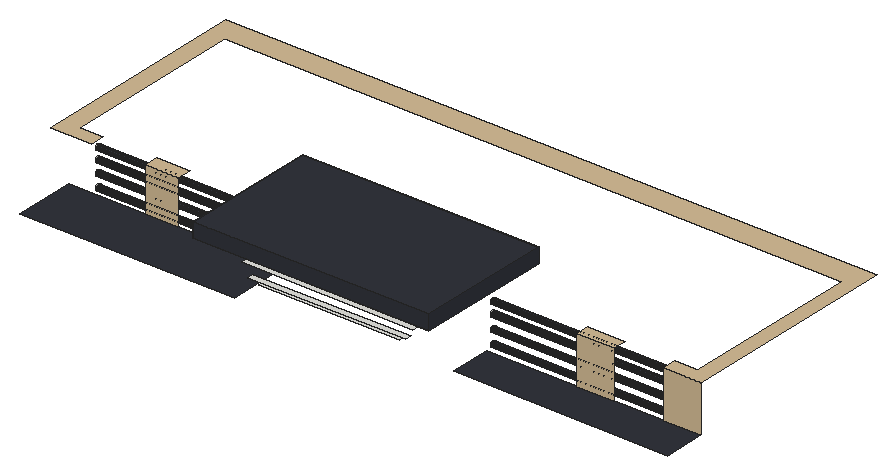
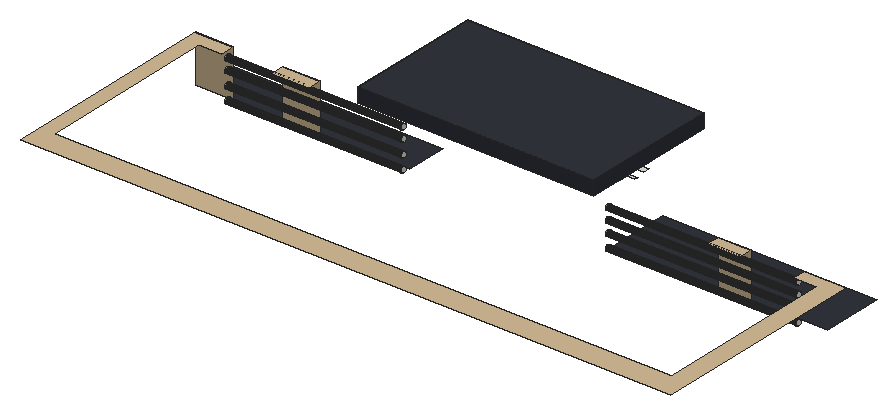
# SketchUp Ruby script. Lengths in inches.
U = 1.inch
M = Sketchup.active_model
def pt(a) = Geom::Point3d.new(a.map { |v| v * U })
def face(e, loops, mat)
  f = e.add_face(loops[0].map { |a| pt(a) })
  loops[1..].each { |l| e.add_face(l.map { |a| pt(a) }).erase! }
  f.material = f.back_material = mat if mat
  f
end
# faces: each face lists its corners as indices into pts; further lists are holes
def faces(e, pts, list, mat = nil) = list.each { |f| face(e, (f[0].is_a?(Array) ? f : [f]).map { |l| l.map { |i| pts[i] } }, mat) }
# xy, xz, yz: faces in a plane at the given z, y or x. An outline is a flat list of corners, or four numbers for a rectangle; further outlines are holes
def ring(l) = l.size == 4 ? [[l[0], l[1]], [l[2], l[1]], [l[2], l[3]], [l[0], l[3]]] : l.each_slice(2).to_a
def flat(e, list, mat, &to3) = list.each { |f| face(e, (f[0].is_a?(Array) ? f : [f]).map { |l| ring(l).map { |u, v| to3.(u, v) } }, mat) }
def xy(e, z, list, mat = nil) = flat(e, list, mat) { |x, y| [x, y, z] }
def xz(e, y, list, mat = nil) = flat(e, list, mat) { |x, z| [x, y, z] }
def yz(e, x, list, mat = nil) = flat(e, list, mat) { |y, z| [x, y, z] }
def lines(e, pts, list) = list.each { |a, b| e.add_line(pt(pts[a]), pt(pts[b])) }
# prism: a flat outline (further loops are holes) pulled along v
def prism(e, loops, v, mat = nil)
  f = face(e, loops, mat); d = Geom::Vector3d.new(v.map { |x| x * U })
  f.pushpull(f.normal.samedirection?(d) ? d.length : -d.length)
end
def box(e, o, s, mat = nil) = prism(e, [[o, [o[0] + s[0], o[1], o[2]], [o[0] + s[0], o[1] + s[1], o[2]], [o[0], o[1] + s[1], o[2]]]], [0, 0, s[2]], mat)
def at(x, y, z, deg = 0) = Geom::Transformation.translation(pt([x, y, z])) * Geom::Transformation.rotation(ORIGIN, Z_AXIS, deg.degrees)
def axes(o, x, y, z) = Geom::Transformation.new([*x, 0, *y, 0, *z, 0, *pt(o).to_a, 1])
def part(name) = M.definitions.add(name)
# library, detail: a bought-in or finely detailed component or shape, given as its bounding box
def library(name, o, s) = part(name).tap { |d| box(d.entities, o, s) }
def detail(e, o, s) = box(e.add_group.entities, o, s)
def put(e, d, t, mat = nil) = e.add_instance(d, t).tap { |i| i.material = mat if mat }
def group(e, t, mat = nil) = e.add_group.tap { |g| g.transformation = t; g.material = mat if mat }.entities
root = M.entities
M.materials.add("[Formica Beige]").color = [211, 187, 149]
M.materials.add("[Formica Laminate Dark]").color = [50, 53, 60]
xy(root,263.9375,[[280.13,426.61,409.38,451.42]],"[Formica Laminate Dark]")
xy(root,265.6875,[[28.78,414.84,157.59,451.42]],"[Formica Laminate Dark]")
xy(root,279.69,[[174.14,412.53,259.2,414.84]])
xy(root,284,[[170.76,408.78,265.76,412.53]])
xy(root,290.79,[[166.89,408.78,270.12,414.84]])
xy(root,292.375,[[17.625,451.42,42.4,451.42,42.4,459.89,28.78,459.89,28.78,568.57,400.54,568.57,400.54,459.89,386.6,459.89,386.6,451.42,409.38,451.42,409.38,583.14,17.625,583.14],[74.87,451.42,94.58,459.89],[334.34,451.42,356.76,459.89]],"[Formica Beige]")
xy(root,305.4375,[[157.59,414.84,280.13,463.02]])
xy(root,305.4375,[[150.71,392.47,292.81,414.84],[150.71,414.84,157.59,454.92],[280.13,414.84,292.81,454.92],[150.71,454.92,157.59,463.02],[280.13,454.92,292.81,474.77],
  [150.71,463.02,280.13,474.77]],"[Formica Laminate Dark]")
xy(root,314.125,[[150.71,392.47,292.81,474.77]],"[Formica Laminate Dark]")
xz(root,392.47,[[150.71,305.4375,292.81,314.125]],"[Formica Laminate Dark]")
xz(root,451.42,[[334.34,263.9375,356.76,292.375],[386.6,263.9375,409.38,292.375],[74.87,265.6875,94.58,292.375]],"[Formica Beige]")
xz(root,474.77,[[150.71,305.4375,292.81,314.125]],"[Formica Laminate Dark]")
yz(root,42.4,[[456.03,265.2,455.63,265.25,455.25,265.41,454.93,265.66,454.68,265.98,454.52,266.36,454.47,266.76,454.52,267.17,454.68,267.54,454.93,267.87,455.25,268.11,455.63,268.27,456.03,268.32,456.4375,268.27,456.8125,268.11,457.14,267.87,457.39,267.54,457.54,267.17,457.6,266.76,457.54,266.36,457.39,265.98,457.14,265.66,456.8125,265.41,456.4375,265.25],[456.03,273.07,455.63,273.125,455.25,273.28,454.93,273.53,454.68,273.85,454.52,274.23,454.47,274.64,454.52,275.04,454.68,275.42,454.93,275.74,455.25,275.99,455.63,276.15,456.03,276.2,456.4375,276.15,456.8125,275.99,457.14,275.74,457.39,275.42,457.54,275.04,457.6,274.64,457.54,274.23,457.39,273.85,457.14,273.53,456.8125,273.28,456.4375,273.125],[456.03,280.26,455.63,280.3125,455.25,280.47,454.93,280.72,454.68,281.04,454.52,281.42,454.47,281.82,454.52,282.23,454.68,282.6,454.93,282.93,455.25,283.18,455.63,283.33,456.03,283.39,456.4375,283.33,456.8125,283.18,457.14,282.93,457.39,282.6,457.54,282.23,457.6,281.82,457.54,281.42,457.39,281.04,457.14,280.72,456.8125,280.47,456.4375,280.3125],[456.03,287.07,455.63,287.125,455.25,287.28,454.93,287.53,454.68,287.85,454.52,288.23,454.47,288.64,454.52,289.04,454.68,289.42,454.93,289.74,455.25,289.99,455.63,290.15,456.03,290.2,456.4375,290.15,456.8125,289.99,457.14,289.74,457.39,289.42,457.54,289.04,457.6,288.64,457.54,288.23,457.39,287.85,457.14,287.53,456.8125,287.28,456.4375,287.125]])
yz(root,150.71,[[392.47,305.4375,474.77,314.125]],"[Formica Laminate Dark]")
yz(root,157.59,[[456.03,265.2,456.4375,265.25,456.8125,265.41,457.14,265.66,457.39,265.98,457.54,266.36,457.6,266.76,457.54,267.17,457.39,267.54,457.14,267.87,456.8125,268.11,456.4375,268.27,456.03,268.32,455.63,268.27,455.25,268.11,454.93,267.87,454.92,267.86,454.92,265.66,454.93,265.66,455.25,265.41,455.63,265.25],[454.92,265.66,454.92,267.86,454.68,267.54,454.52,267.17,454.47,266.76,454.52,266.36,454.68,265.98],[456.03,273.07,456.4375,273.125,456.8125,273.28,457.14,273.53,457.39,273.85,457.54,274.23,457.6,274.64,457.54,275.04,457.39,275.42,457.14,275.74,456.8125,275.99,456.4375,276.15,456.03,276.2,455.63,276.15,455.25,275.99,454.93,275.74,454.92,275.73,454.92,273.54,454.93,273.53,455.25,273.28,455.63,273.125],[454.92,273.54,454.92,275.73,454.68,275.42,454.52,275.04,454.47,274.64,454.52,274.23,454.68,273.85],[456.03,280.26,456.4375,280.3125,456.8125,280.47,457.14,280.72,457.39,281.04,457.54,281.42,457.6,281.82,457.54,282.23,457.39,282.6,457.14,282.93,456.8125,283.18,456.4375,283.33,456.03,283.39,455.63,283.33,455.25,283.18,454.93,282.93,454.92,282.92,454.92,280.73,454.93,280.72,455.25,280.47,455.63,280.3125],
  [454.92,280.73,454.92,282.92,454.68,282.6,454.52,282.23,454.47,281.82,454.52,281.42,454.68,281.04],[456.03,287.07,456.4375,287.125,456.8125,287.28,457.14,287.53,457.39,287.85,457.54,288.23,457.6,288.64,457.54,289.04,457.39,289.42,457.14,289.74,456.8125,289.99,456.4375,290.15,456.03,290.2,455.63,290.15,455.25,289.99,454.93,289.74,454.92,289.73,454.92,287.54,454.93,287.53,455.25,287.28,455.63,287.125],[454.92,287.54,454.92,289.73,454.68,289.42,454.52,289.04,454.47,288.64,454.52,288.23,454.68,287.85]])
yz(root,280.13,[[456.12,264.23,455.71,264.28,455.33,264.44,455.01,264.68,454.92,264.8,454.92,266.78,455.01,266.89,455.33,267.14,455.71,267.3,456.12,267.35,456.52,267.3,456.9,267.14,457.22,266.89,457.47,266.57,457.625,266.19,457.68,265.79,457.625,265.38,457.47,265.01,457.22,264.68,456.9,264.44,456.52,264.28],[454.92,264.8,454.76,265.01,454.61,265.38,454.55,265.79,454.61,266.19,454.76,266.57,454.92,266.78],[456.12,272.29,455.71,272.34,455.33,272.5,455.01,272.75,454.92,272.86,454.92,274.84,455.01,274.96,455.33,275.2,455.71,275.36,456.12,275.41,456.52,275.36,456.9,275.2,457.22,274.96,457.47,274.63,457.625,274.26,457.68,273.85,457.625,273.45,457.47,273.07,457.22,272.75,456.9,272.5,456.52,272.34],[454.92,272.86,454.76,273.07,454.61,273.45,454.55,273.85,454.61,274.26,454.76,274.63,454.92,274.84],[456.12,280.66,455.71,280.72,455.33,280.87,455.01,281.12,454.92,281.24,454.92,283.21,455.01,283.33,455.33,283.58,455.71,283.74,456.12,283.79,456.52,283.74,456.9,283.58,457.22,283.33,457.47,283.01,457.625,282.63,457.68,282.23,457.625,281.82,457.47,281.44,457.22,281.12,456.9,280.87,456.52,280.72],
  [454.92,281.24,454.76,281.44,454.61,281.82,454.55,282.23,454.61,282.63,454.76,283.01,454.92,283.21],[456.12,287.41,455.71,287.47,455.33,287.62,455.01,287.87,454.92,287.99,454.92,289.96,455.01,290.08,455.33,290.33,455.71,290.49,456.12,290.54,456.52,290.49,456.9,290.33,457.22,290.08,457.47,289.76,457.625,289.38,457.68,288.98,457.625,288.57,457.47,288.19,457.22,287.87,456.9,287.62,456.52,287.47],[454.92,287.99,454.76,288.19,454.61,288.57,454.55,288.98,454.61,289.38,454.76,289.76,454.92,289.96]])
yz(root,292.81,[[392.47,305.4375,474.77,314.125]],"[Formica Laminate Dark]")
yz(root,386.6,[[456.12,264.23,456.52,264.28,456.9,264.44,457.22,264.68,457.47,265.01,457.625,265.38,457.68,265.79,457.625,266.19,457.47,266.57,457.22,266.89,456.9,267.14,456.52,267.3,456.12,267.35,455.71,267.3,455.33,267.14,455.01,266.89,454.76,266.57,454.61,266.19,454.55,265.79,454.61,265.38,454.76,265.01,455.01,264.68,455.33,264.44,455.71,264.28],[456.12,272.29,456.52,272.34,456.9,272.5,457.22,272.75,457.47,273.07,457.625,273.45,457.68,273.85,457.625,274.26,457.47,274.63,457.22,274.96,456.9,275.2,456.52,275.36,456.12,275.41,455.71,275.36,455.33,275.2,455.01,274.96,454.76,274.63,454.61,274.26,454.55,273.85,454.61,273.45,454.76,273.07,455.01,272.75,455.33,272.5,455.71,272.34],[456.12,280.66,456.52,280.72,456.9,280.87,457.22,281.12,457.47,281.44,457.625,281.82,457.68,282.23,457.625,282.63,457.47,283.01,457.22,283.33,456.9,283.58,456.52,283.74,456.12,283.79,455.71,283.74,455.33,283.58,455.01,283.33,454.76,283.01,454.61,282.63,454.55,282.23,454.61,281.82,454.76,281.44,455.01,281.12,455.33,280.87,455.71,280.72],[456.12,287.41,456.52,287.47,456.9,287.62,457.22,287.87,457.47,288.19,457.625,288.57,457.68,288.98,457.625,289.38,457.47,289.76,457.22,290.08,456.9,290.33,456.52,290.49,456.12,290.54,455.71,290.49,455.33,290.33,455.01,290.08,454.76,289.76,454.61,289.38,454.55,288.98,454.61,288.57,454.76,288.19,455.01,287.87,455.33,287.62,455.71,287.47]])
p = [[386.6,456.12,264.23],[386.6,455.71,264.28],[280.13,455.71,264.28],[280.13,456.12,264.23],[386.6,456.52,264.28],[280.13,456.52,264.28],
  [386.6,455.33,264.44],[280.13,455.33,264.44],[386.6,456.9,264.44],[280.13,456.9,264.44],[386.6,455.01,264.68],[280.13,455.01,264.68],
  [386.6,457.22,264.68],[280.13,457.22,264.68],[386.6,454.76,265.01],[280.13,454.76,265.01],[280.13,454.92,264.8],[386.6,457.47,265.01],
  [280.13,457.47,265.01],[386.6,454.61,265.38],[280.13,454.61,265.38],[386.6,457.625,265.38],[280.13,457.625,265.38],[42.4,455.63,265.25],
  [42.4,456.03,265.2],[157.59,456.03,265.2],[157.59,455.63,265.25],[42.4,456.4375,265.25],[157.59,456.4375,265.25],[42.4,455.25,265.41],
  [157.59,455.25,265.41],[42.4,456.8125,265.41],[157.59,456.8125,265.41],[386.6,454.55,265.79],[280.13,454.55,265.79],[42.4,454.93,265.66],
  [157.59,454.93,265.66],[42.4,457.14,265.66],[157.59,457.14,265.66],[386.6,457.68,265.79],[280.13,457.68,265.79],[42.4,454.68,265.98],
  [157.59,454.92,265.66],[157.59,454.68,265.98],[42.4,457.39,265.98],[157.59,457.39,265.98],[386.6,454.61,266.19],[280.13,454.61,266.19],
  [386.6,457.625,266.19],[280.13,457.625,266.19],[42.4,454.52,266.36],[157.59,454.52,266.36],[42.4,457.54,266.36],[157.59,457.54,266.36],
  [386.6,454.76,266.57],[280.13,454.76,266.57],[386.6,457.47,266.57],[280.13,457.47,266.57],[42.4,454.47,266.76],[157.59,454.47,266.76],
  [42.4,457.6,266.76],[157.59,457.6,266.76],[386.6,455.01,266.89],[280.13,455.01,266.89],[280.13,454.92,266.78],[386.6,457.22,266.89],
  [280.13,457.22,266.89],[42.4,454.52,267.17],[157.59,454.52,267.17],[42.4,457.54,267.17],[157.59,457.54,267.17],[386.6,455.33,267.14],
  [280.13,455.33,267.14],[386.6,456.9,267.14],[280.13,456.9,267.14],[386.6,455.71,267.3],[280.13,455.71,267.3],[386.6,456.52,267.3],
  [280.13,456.52,267.3],[42.4,454.68,267.54],[157.59,454.68,267.54],[42.4,457.39,267.54],[157.59,457.39,267.54],[386.6,456.12,267.35],
  [280.13,456.12,267.35],[42.4,454.93,267.87],[157.59,454.92,267.86],[157.59,454.93,267.87],[42.4,457.14,267.87],[157.59,457.14,267.87],
  [42.4,455.25,268.11],[157.59,455.25,268.11],[42.4,456.8125,268.11],[157.59,456.8125,268.11],[42.4,455.63,268.27],[157.59,455.63,268.27],
  [42.4,456.4375,268.27],[157.59,456.4375,268.27],[42.4,456.03,268.32],[157.59,456.03,268.32],[386.6,455.71,272.34],[386.6,455.33,272.5],
  [280.13,455.33,272.5],[280.13,455.71,272.34],[386.6,456.12,272.29],[280.13,456.12,272.29],[386.6,456.52,272.34],[280.13,456.52,272.34],
  [386.6,456.9,272.5],[280.13,456.9,272.5],[386.6,455.01,272.75],[280.13,455.01,272.75],[386.6,457.22,272.75],[280.13,457.22,272.75],
  [386.6,454.76,273.07],[280.13,454.76,273.07],[280.13,454.92,272.86],[386.6,457.47,273.07],[280.13,457.47,273.07],[386.6,454.61,273.45],
  [280.13,454.61,273.45],[42.4,455.25,273.28],[42.4,455.63,273.125],[157.59,455.63,273.125],[157.59,455.25,273.28],[42.4,456.03,273.07],
  [157.59,456.03,273.07],[42.4,456.4375,273.125],[157.59,456.4375,273.125],[42.4,456.8125,273.28],[157.59,456.8125,273.28],[386.6,457.625,273.45],
  [280.13,457.625,273.45],[42.4,454.93,273.53],[157.59,454.93,273.53],[42.4,457.14,273.53],[157.59,457.14,273.53],[386.6,454.55,273.85],
  [280.13,454.55,273.85],[386.6,457.68,273.85],[280.13,457.68,273.85],[42.4,454.68,273.85],[157.59,454.92,273.54],[157.59,454.68,273.85],
  [42.4,457.39,273.85],[157.59,457.39,273.85],[42.4,454.52,274.23],[157.59,454.52,274.23],[386.6,454.61,274.26],[280.13,454.61,274.26],
  [42.4,457.54,274.23],[157.59,457.54,274.23],[386.6,457.625,274.26],[280.13,457.625,274.26],[42.4,454.47,274.64],[157.59,454.47,274.64],
  [42.4,457.6,274.64],[157.59,457.6,274.64],[386.6,454.76,274.63],[280.13,454.76,274.63],[386.6,457.47,274.63],[280.13,457.47,274.63],
  [42.4,454.52,275.04],[157.59,454.52,275.04],[386.6,455.01,274.96],[280.13,455.01,274.96],[280.13,454.92,274.84],[386.6,457.22,274.96],
  [280.13,457.22,274.96],[42.4,457.54,275.04],[157.59,457.54,275.04],[42.4,454.68,275.42],[157.59,454.68,275.42],[386.6,455.33,275.2],
  [280.13,455.33,275.2],[386.6,456.9,275.2],[280.13,456.9,275.2],[42.4,457.39,275.42],[157.59,457.39,275.42],[386.6,455.71,275.36],
  [280.13,455.71,275.36],[386.6,456.52,275.36],[280.13,456.52,275.36],[42.4,454.93,275.74],[157.59,454.92,275.73],[157.59,454.93,275.74],
  [386.6,456.12,275.41],[280.13,456.12,275.41],[42.4,457.14,275.74],[157.59,457.14,275.74],[42.4,455.25,275.99],[157.59,455.25,275.99],
  [42.4,456.8125,275.99],[157.59,456.8125,275.99],[42.4,455.63,276.15],[157.59,455.63,276.15],[42.4,456.4375,276.15],[157.59,456.4375,276.15],
  [42.4,456.03,276.2],[157.59,456.03,276.2],[42.4,455.25,280.47],[42.4,455.63,280.3125],[157.59,455.63,280.3125],[157.59,455.25,280.47],
  [42.4,456.03,280.26],[157.59,456.03,280.26],[42.4,456.4375,280.3125],[157.59,456.4375,280.3125],[42.4,456.8125,280.47],[157.59,456.8125,280.47],
  [42.4,454.93,280.72],[157.59,454.93,280.72],[42.4,457.14,280.72],[157.59,457.14,280.72],[42.4,454.68,281.04],[157.59,454.92,280.73],
  [157.59,454.68,281.04],[386.6,455.71,280.72],[386.6,455.33,280.87],[280.13,455.33,280.87],[280.13,455.71,280.72],[386.6,456.12,280.66],
  [280.13,456.12,280.66],[386.6,456.52,280.72],[280.13,456.52,280.72],[386.6,456.9,280.87],[280.13,456.9,280.87],[42.4,457.39,281.04],
  [157.59,457.39,281.04],[386.6,455.01,281.12],[280.13,455.01,281.12],[386.6,457.22,281.12],[280.13,457.22,281.12],[42.4,454.52,281.42],
  [157.59,454.52,281.42],[42.4,457.54,281.42],[157.59,457.54,281.42],[386.6,454.76,281.44],[280.13,454.76,281.44],[280.13,454.92,281.24],
  [386.6,457.47,281.44],[280.13,457.47,281.44],[42.4,454.47,281.82],[157.59,454.47,281.82],[386.6,454.61,281.82],[280.13,454.61,281.82],
  [42.4,457.6,281.82],[157.59,457.6,281.82],[386.6,457.625,281.82],[280.13,457.625,281.82],[42.4,454.52,282.23],[157.59,454.52,282.23],
  [386.6,454.55,282.23],[280.13,454.55,282.23],[42.4,457.54,282.23],[157.59,457.54,282.23],[386.6,457.68,282.23],[280.13,457.68,282.23],
  [42.4,454.68,282.6],[157.59,454.68,282.6],[386.6,454.61,282.63],[280.13,454.61,282.63],[42.4,457.39,282.6],[157.59,457.39,282.6],
  [386.6,457.625,282.63],[280.13,457.625,282.63],[386.6,454.76,283.01],[280.13,454.76,283.01],[42.4,454.93,282.93],[157.59,454.92,282.92],
  [157.59,454.93,282.93],[42.4,457.14,282.93],[157.59,457.14,282.93],[386.6,457.47,283.01],[280.13,457.47,283.01],[42.4,455.25,283.18],
  [157.59,455.25,283.18],[42.4,456.8125,283.18],[157.59,456.8125,283.18],[386.6,455.01,283.33],[280.13,455.01,283.33],[280.13,454.92,283.21],
  [386.6,457.22,283.33],[280.13,457.22,283.33],[42.4,455.63,283.33],[157.59,455.63,283.33],[42.4,456.4375,283.33],[157.59,456.4375,283.33],
  [386.6,455.33,283.58],[280.13,455.33,283.58],[42.4,456.03,283.39],[157.59,456.03,283.39],[386.6,456.9,283.58],[280.13,456.9,283.58],
  [386.6,455.71,283.74],[280.13,455.71,283.74],[386.6,456.52,283.74],[280.13,456.52,283.74],[386.6,456.12,283.79],[280.13,456.12,283.79],
  [42.4,455.25,287.28],[42.4,455.63,287.125],[157.59,455.63,287.125],[157.59,455.25,287.28],[42.4,456.03,287.07],[157.59,456.03,287.07],
  [42.4,456.4375,287.125],[157.59,456.4375,287.125],[42.4,456.8125,287.28],[157.59,456.8125,287.28],[42.4,454.93,287.53],[157.59,454.93,287.53],
  [42.4,457.14,287.53],[157.59,457.14,287.53],[386.6,456.12,287.41],[386.6,455.71,287.47],[280.13,455.71,287.47],[280.13,456.12,287.41],
  [386.6,456.52,287.47],[280.13,456.52,287.47],[42.4,454.68,287.85],[157.59,454.92,287.54],[157.59,454.68,287.85],[386.6,455.33,287.62],
  [280.13,455.33,287.62],[386.6,456.9,287.62],[280.13,456.9,287.62],[42.4,457.39,287.85],[157.59,457.39,287.85],[386.6,455.01,287.87],
  [280.13,455.01,287.87],[386.6,457.22,287.87],[280.13,457.22,287.87],[42.4,454.52,288.23],[157.59,454.52,288.23],[386.6,454.76,288.19],
  [280.13,454.76,288.19],[280.13,454.92,287.99],[386.6,457.47,288.19],[280.13,457.47,288.19],[42.4,457.54,288.23],[157.59,457.54,288.23],
  [42.4,454.47,288.64],[157.59,454.47,288.64],[386.6,454.61,288.57],[280.13,454.61,288.57],[42.4,457.6,288.64],[157.59,457.6,288.64],
  [386.6,457.625,288.57],[280.13,457.625,288.57],[42.4,454.52,289.04],[157.59,454.52,289.04],[386.6,454.55,288.98],[280.13,454.55,288.98],
  [42.4,457.54,289.04],[157.59,457.54,289.04],[386.6,457.68,288.98],[280.13,457.68,288.98],[42.4,454.68,289.42],[157.59,454.68,289.42],
  [386.6,454.61,289.38],[280.13,454.61,289.38],[42.4,457.39,289.42],[157.59,457.39,289.42],[386.6,457.625,289.38],[280.13,457.625,289.38],
  [386.6,454.76,289.76],[280.13,454.76,289.76],[42.4,454.93,289.74],[157.59,454.92,289.73],[157.59,454.93,289.74],[42.4,457.14,289.74],
  [157.59,457.14,289.74],[386.6,457.47,289.76],[280.13,457.47,289.76],[42.4,455.25,289.99],[157.59,455.25,289.99],[42.4,456.8125,289.99],
  [157.59,456.8125,289.99],[386.6,455.01,290.08],[280.13,455.01,290.08],[280.13,454.92,289.96],[386.6,457.22,290.08],[280.13,457.22,290.08],
  [42.4,455.63,290.15],[157.59,455.63,290.15],[42.4,456.4375,290.15],[157.59,456.4375,290.15],[386.6,455.33,290.33],[280.13,455.33,290.33],
  [42.4,456.03,290.2],[157.59,456.03,290.2],[386.6,456.9,290.33],[280.13,456.9,290.33],[386.6,455.71,290.49],[280.13,455.71,290.49],
  [386.6,456.52,290.49],[280.13,456.52,290.49],[386.6,456.12,290.54],[280.13,456.12,290.54]]
faces(root,p,[[0,1,2,3],[4,0,3,5],[1,6,7,2],[8,4,5,9],[6,10,11,7],[12,8,9,13],[10,14,15,16,11],[17,12,13,18],
  [14,19,20,15],[21,17,18,22],[23,24,25,26],[24,27,28,25],[29,23,26,30],[27,31,32,28],[19,33,34,20],[35,29,30,36],
  [31,37,38,32],[39,21,22,40],[41,35,36,42,43],[37,44,45,38],[33,46,47,34],[48,39,40,49],[50,41,43,51],[44,52,53,45],
  [46,54,55,47],[56,48,49,57],[58,50,51,59],[52,60,61,53],[54,62,63,64,55],[65,56,57,66],[67,58,59,68],[60,69,70,61],
  [62,71,72,63],[73,65,66,74],[71,75,76,72],[77,73,74,78],[79,67,68,80],[69,81,82,70],[75,83,84,76],[83,77,78,84],
  [85,79,80,86,87],[81,88,89,82],[90,85,87,91],[88,92,93,89],[94,90,91,95],[92,96,97,93],[98,94,95,99],[96,98,99,97],
  [100,101,102,103],[104,100,103,105],[106,104,105,107],[108,106,107,109],[101,110,111,102],[112,108,109,113],[110,114,115,116,111],[117,112,113,118],
  [114,119,120,115],[121,122,123,124],[122,125,126,123],[125,127,128,126],[127,129,130,128],[131,117,118,132],[133,121,124,134],[129,135,136,130],
  [119,137,138,120],[139,131,132,140],[141,133,134,142,143],[135,144,145,136],[146,141,143,147],[137,148,149,138],[144,150,151,145],[152,139,140,153],
  [154,146,147,155],[150,156,157,151],[148,158,159,149],[160,152,153,161],[162,154,155,163],[158,164,165,166,159],[167,160,161,168],[156,169,170,157],
  [171,162,163,172],[164,173,174,165],[175,167,168,176],[169,177,178,170],[173,179,180,174],[181,175,176,182],[183,171,172,184,185],[179,186,187,180],
  [186,181,182,187],[177,188,189,178],[190,183,185,191],[188,192,193,189],[194,190,191,195],[192,196,197,193],[198,194,195,199],[196,198,199,197],
  [200,201,202,203],[201,204,205,202],[204,206,207,205],[206,208,209,207],[210,200,203,211],[208,212,213,209],[214,210,211,215,216],[217,218,219,220],
  [221,217,220,222],[223,221,222,224],[225,223,224,226],[212,227,228,213],[218,229,230,219],[231,225,226,232],[233,214,216,234],[227,235,236,228],
  [229,237,238,239,230],[240,231,232,241],[242,233,234,243],[237,244,245,238],[235,246,247,236],[248,240,241,249],[250,242,243,251],[244,252,253,245],
  [246,254,255,247],[256,248,249,257],[258,250,251,259],[252,260,261,253],[254,262,263,255],[264,256,257,265],[260,266,267,261],[268,258,259,269,270],
  [262,271,272,263],[273,264,265,274],[275,268,270,276],[271,277,278,272],[266,279,280,281,267],[282,273,274,283],[284,275,276,285],[277,286,287,278],
  [279,288,289,280],[290,284,285,291],[286,290,291,287],[292,282,283,293],[288,294,295,289],[296,292,293,297],[294,298,299,295],[298,296,297,299],
  [300,301,302,303],[301,304,305,302],[304,306,307,305],[306,308,309,307],[310,300,303,311],[308,312,313,309],[314,315,316,317],[318,314,317,319],
  [320,310,311,321,322],[315,323,324,316],[325,318,319,326],[312,327,328,313],[323,329,330,324],[331,325,326,332],[333,320,322,334],[329,335,336,337,330],
  [338,331,332,339],[327,340,341,328],[342,333,334,343],[335,344,345,336],[340,346,347,341],[348,338,339,349],[350,342,343,351],[344,352,353,345],
  [346,354,355,347],[356,348,349,357],[358,350,351,359],[352,360,361,353],[354,362,363,355],[364,356,357,365],[360,366,367,361],[368,358,359,369,370],
  [362,371,372,363],[373,364,365,374],[375,368,370,376],[371,377,378,372],[366,379,380,381,367],[382,373,374,383],[384,375,376,385],[377,386,387,378],
  [379,388,389,380],[390,384,385,391],[386,390,391,387],[392,382,383,393],[388,394,395,389],[396,392,393,397],[394,398,399,395],[398,396,397,399]],"[Formica Laminate Dark]")
